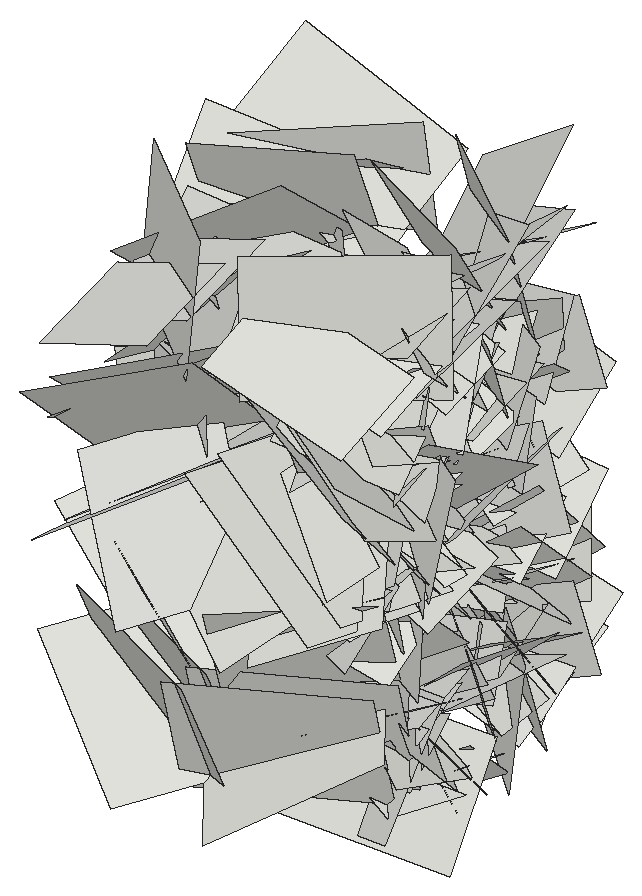
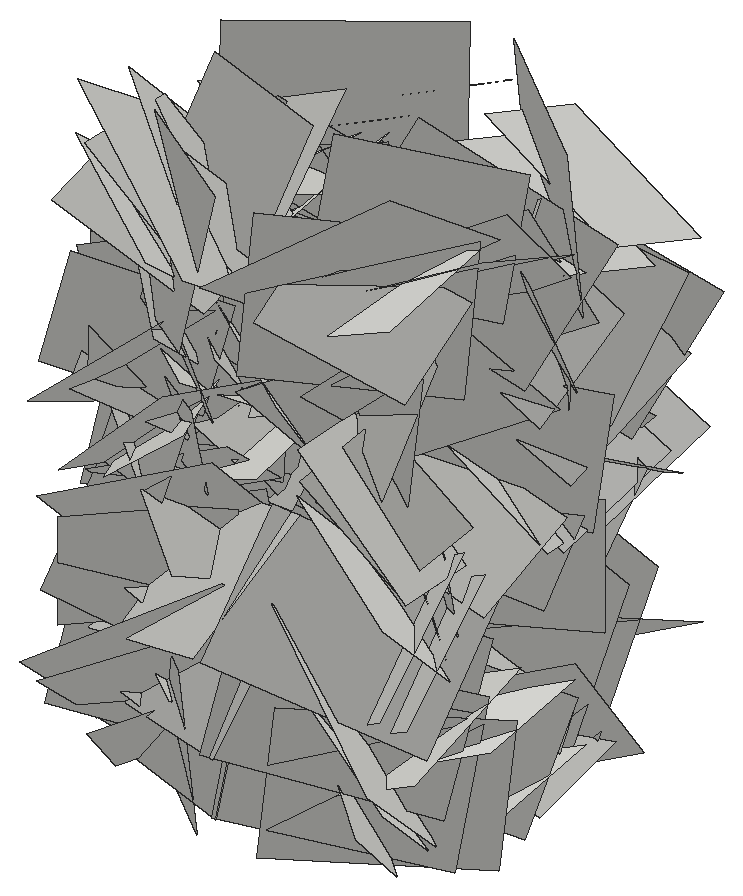
# SketchUp Ruby script. Lengths in inches.
U = 1.inch
M = Sketchup.active_model
def pt(a) = Geom::Point3d.new(a.map { |v| v * U })
def face(e, loops, mat)
  f = e.add_face(loops[0].map { |a| pt(a) })
  loops[1..].each { |l| e.add_face(l.map { |a| pt(a) }).erase! }
  f.material = f.back_material = mat if mat
  f
end
# faces: each face lists its corners as indices into pts; further lists are holes
def faces(e, pts, list, mat = nil) = list.each { |f| face(e, (f[0].is_a?(Array) ? f : [f]).map { |l| l.map { |i| pts[i] } }, mat) }
# xy, xz, yz: faces in a plane at the given z, y or x. An outline is a flat list of corners, or four numbers for a rectangle; further outlines are holes
def ring(l) = l.size == 4 ? [[l[0], l[1]], [l[2], l[1]], [l[2], l[3]], [l[0], l[3]]] : l.each_slice(2).to_a
def flat(e, list, mat, &to3) = list.each { |f| face(e, (f[0].is_a?(Array) ? f : [f]).map { |l| ring(l).map { |u, v| to3.(u, v) } }, mat) }
def xy(e, z, list, mat = nil) = flat(e, list, mat) { |x, y| [x, y, z] }
def xz(e, y, list, mat = nil) = flat(e, list, mat) { |x, z| [x, y, z] }
def yz(e, x, list, mat = nil) = flat(e, list, mat) { |y, z| [x, y, z] }
def lines(e, pts, list) = list.each { |a, b| e.add_line(pt(pts[a]), pt(pts[b])) }
# prism: a flat outline (further loops are holes) pulled along v
def prism(e, loops, v, mat = nil)
  f = face(e, loops, mat); d = Geom::Vector3d.new(v.map { |x| x * U })
  f.pushpull(f.normal.samedirection?(d) ? d.length : -d.length)
end
def box(e, o, s, mat = nil) = prism(e, [[o, [o[0] + s[0], o[1], o[2]], [o[0] + s[0], o[1] + s[1], o[2]], [o[0], o[1] + s[1], o[2]]]], [0, 0, s[2]], mat)
def at(x, y, z, deg = 0) = Geom::Transformation.translation(pt([x, y, z])) * Geom::Transformation.rotation(ORIGIN, Z_AXIS, deg.degrees)
def axes(o, x, y, z) = Geom::Transformation.new([*x, 0, *y, 0, *z, 0, *pt(o).to_a, 1])
def part(name) = M.definitions.add(name)
# library, detail: a bought-in or finely detailed component or shape, given as its bounding box
def library(name, o, s) = part(name).tap { |d| box(d.entities, o, s) }
def detail(e, o, s) = box(e.add_group.entities, o, s)
def put(e, d, t, mat = nil) = e.add_instance(d, t).tap { |i| i.material = mat if mat }
def group(e, t, mat = nil) = e.add_group.tap { |g| g.transformation = t; g.material = mat if mat }.entities
root = M.entities
c1 = part("Component\#6")
p = [[0.01,0,0],[0,3.24,4.54],[4.32,3.24,4.54],[4.33,0,0]]
faces(c1.entities,p,[[0,1,2,3]])
put(root,c1,axes([14.53,133.2,0.29],[-0.16868,0.00753,1.30134],[-0.16064,1.302,-0.02607],[1.37005,0.15359,0.15716]))
put(root,c1,axes([18.5,127.28,0.51],[0.04452,-0.40985,0.5808],[0.07759,0.58122,0.40485],[-0.7495,0.03582,0.07641]))
put(root,c1,axes([14.53,129.68,16.21],[0.16446,-0.17941,-0.82447],[0.07006,-0.83314,0.19373],[0.89165,0.09856,0.13685]))
put(root,c1,axes([18.5,134.26,15.51],[0.13639,0.72841,-0.25059],[0.07067,-0.26364,-0.7321],[-0.81346,0.09922,-0.10562]))
put(root,c1,axes([14.53,128.87,2.92],[0.01411,0.95221,-0.19006],[0.11482,-0.19035,-0.94606],[1.02282,0.00823,0.10882]))
put(root,c1,axes([14.53,138.97,11.375],[-0.02639,-0.72989,-0.72722],[0.07911,-0.7268,0.72691],[1.08928,0.0351,-0.07041]))
put(root,c1,axes([14.53,131.74,20.5625],[-0.11289,-0.41624,-1.03402],[0.06809,-1.03929,0.41174],[1.17957,0.02016,-0.12272]))
put(root,c1,axes([18.5,131.9,7.66],[0.03371,0.19161,0.61883],[0.06203,0.6162,-0.1938],[-0.68388,0.06533,0.01292]))
put(root,c1,axes([14.53,134.95,12.42],[0.03363,0.92541,-1.00089],[-0.39451,-0.95725,-0.89685],[1.39004,-0.29406,-0.23032]))
put(root,c1,axes([18.5,131.8,8.64],[0.08497,0.05507,0.67491],[0.04101,0.67814,-0.05993],[-0.71661,0.04534,0.0766]))
put(root,c1,axes([14.53,137.89,18.97],[0.02244,-0.79516,0.48934],[0.22215,0.48102,0.77258],[0.96443,-0.0923,-0.18934]))
put(root,c1,axes([14.53,137.87,11.82],[0.23548,-0.98581,-0.19043],[-0.17104,-0.22756,0.98976],[1.05044,0.18394,0.20385]))
put(root,c1,axes([14.53,129.625,19.87],[-0.14331,0.9196,0.97349],[-0.15794,0.96203,-0.92947],[1.41069,0.20113,-0.00516]))
put(root,c1,axes([14.53,130.99,8.6],[0.04494,-0.64922,0.68663],[0.20873,0.6783,0.62918],[0.97967,-0.11474,-0.16555]))
put(root,c1,axes([14.53,133.91,11.1875],[-0.02059,0.92356,-0.8814],[-0.20413,-0.87353,-0.91107],[1.33776,-0.11908,-0.15259]))
put(root,c1,axes([14.53,128.56,10.3125],[-0.23413,0.04823,1.24691],[0.1221,1.26168,-0.02839],[1.31707,-0.10839,0.22429]))
put(root,c1,axes([14.53,131.94,16.85],[-0.08825,-0.96476,0.81898],[-0.08011,0.82307,0.9619],[1.33903,-0.01434,0.11152]))
put(root,c1,axes([14.53,131.18,15.16],[0.15294,-1.16278,0.39158],[-0.28955,0.35393,1.15166],[1.26792,0.22109,0.21577]))
put(root,c1,axes([18.5,134.77,2.57],[0.05447,0.40704,0.46107],[0.08155,0.45478,-0.41007],[-0.64681,0.09162,-0.01288]))
put(root,c1,axes([14.53,134.14,22.88],[0.03825,0.99518,-0.25742],[0.13842,-0.25993,-0.98657],[1.08078,-0.00193,0.13547]))
put(root,c1,axes([13.82,124.93,11.12],[0.54058,0.75668,0.32998],[0.30141,0.20311,-0.90522],[0.82148,-0.57246,0.11499]))
put(root,c1,axes([14.53,127.92,6.47],[-0.03611,0.05394,1.13531],[0.09971,1.13206,-0.05096],[1.20066,-0.09239,0.03838]))
put(root,c1,axes([18.5,138.1,17.99],[0.00934,-0.49027,-0.41508],[0.1892,-0.3969,0.47259],[-0.65411,-0.1218,0.13076]))
put(root,c1,axes([14.53,127.69,20.12],[-0.02742,-1.01137,-0.35231],[0.21232,-0.35076,0.99222],[1.1152,0.04191,-0.19757]))
put(root,c1,axes([14.53,130,20.12],[-0.02742,-1.01137,-0.35231],[0.21232,-0.35076,0.99222],[1.1152,0.04191,-0.19757]))
put(root,c1,axes([18.5,129.35,18.22],[0.07955,-0.40219,0.442],[0.06566,0.44831,0.39741],[-0.63004,-0.00406,0.09723]))
put(root,c1,axes([14.53,129.81,24.32],[-0.08615,-0.07511,-1.33483],[-0.12267,-1.33188,0.08199],[1.41184,-0.12031,-0.07433]))
put(root,c1,axes([14.53,131.16,1.32],[0.11103,-1.00768,0.14491],[0.13016,0.15712,1.00381],[1.07125,0.08535,-0.13699]))
put(root,c1,axes([14.53,136.29,19.65],[0.239,0.33681,-1.04778],[-0.13934,-1.05364,-0.36698],[1.15826,-0.19625,0.17205]))
put(root,c1,axes([14.53,129.42,5.47],[-0.26825,1.30607,0.06413],[0.25565,0.11082,-1.30519],[1.36232,0.23638,0.25756]))
put(root,c1,axes([14.53,126.61,12.8],[-0.1414,-0.87971,0.87765],[0.19082,0.8597,0.88908],[1.30331,-0.22132,-0.03495]))
put(root,c1,axes([14.53,133.96,9.66],[0.06967,-1.04066,0.34132],[0.1454,0.34706,1.03175],[1.15177,0.01914,-0.15089]))
put(root,c1,axes([14.53,134.94,17.85],[0.08672,-0.29938,1.1859],[-0.04442,1.18717,0.30259],[1.29573,0.06074,-0.069]))
put(root,c1,axes([14.53,129.48,20.64],[-0.14207,1.22324,0.51937],[0.11373,0.53026,-1.2212],[1.40407,0.08082,0.15147]))
put(root,c1,axes([14.53,129.66,12.47],[-0.1081,-1.2535,0.58167],[-0.00417,0.58351,1.25678],[1.46479,-0.09085,0.0465]))
put(root,c1,axes([14.53,125.82,11.42],[0.20547,0.4933,-0.99975],[0.03886,-1.01702,-0.49472],[1.18108,-0.05236,0.1902]))
put(root,c1,axes([14.53,131.95,0.87],[0.07095,-0.70744,0.83659],[0.30432,0.82019,0.6706],[1.12076,-0.17792,-0.23504]))
put(root,c1,axes([14.53,139.8125,5.82],[0.12038,-0.94885,-0.86303],[-0.08352,-0.86993,0.94607],[1.35702,0.03063,0.13479]))
put(root,c1,axes([14.53,133.04,19.75],[0.14526,-0.49923,0.95494],[0.24012,0.95446,0.46647],[1.11669,-0.1403,-0.22453]))
put(root,c1,axes([14.53,128.24,17.68],[0.22785,0.52614,1.07761],[-0.06777,1.09826,-0.52347],[1.26934,-0.03581,-0.22138]))
put(root,c1,axes([14.53,133.15,22.79],[0.15509,1.06813,0.73269],[-0.10614,0.74447,-1.06531],[1.36888,-0.06329,-0.16562]))
put(root,c1,axes([14.53,132.12,7.08],[-0.00585,1.22451,-0.43101],[0.11167,-0.42917,-1.22063],[1.3715,0.04016,0.09755]))
put(root,c1,axes([14.53,125.99,1.35],[0.00241,0.79041,1.08039],[0.06651,1.07914,-0.78963],[1.41741,-0.05198,0.03522]))
put(root,c1,axes([14.53,127.67,13.74],[0.06329,-0.97705,0.81505],[0.12838,0.8166,0.97005],[1.34259,-0.03203,-0.13118]))
put(root,c1,axes([14.53,137,19.49],[0.23927,-0.1296,-1.18474],[0.04055,-1.20439,0.13904],[1.26266,0.06324,0.22004]))
put(root,c1,axes([14.53,135.39,1.18],[0.01455,-0.40823,1.27358],[0.1801,1.26386,0.40328],[1.40617,-0.15765,-0.06483]))
put(root,c1,axes([14.53,128.0625,10.23],[0.10909,-1.3698,0.20566],[-0.00727,0.20572,1.37363],[1.46824,0.1028,-0.00848]))
put(root,c1,axes([14.53,129.98,10.23],[0.10909,-1.3698,0.20566],[-0.00727,0.20572,1.37363],[1.46824,0.1028,-0.00848]))
put(root,c1,axes([14.53,138.98,4.78],[0.22268,-0.9196,-0.8307],[0.07298,-0.83259,0.9391],[1.31157,0.20246,0.08879]))
put(root,c1,axes([13.36,124.5,5.79],[0.83668,1.07369,0.2523],[0.21003,0.16716,-1.33127],[1.15009,-0.81162,0.05958]))
put(root,c1,axes([14.53,130.78,10.54],[0.24762,-1.26357,-0.1726],[-0.00687,-0.17664,1.28442],[1.3518,0.23056,0.03815]))
put(root,c1,axes([14.53,136.82,5.83],[0.1656,-1.02965,0.80161],[0.14776,0.81588,1.02082],[1.37528,0.03632,-0.2062]))
put(root,c1,axes([14.53,130.15,15.41],[0.24379,0.89731,1.03665],[0.02149,1.04879,-0.91232],[1.45316,-0.16605,-0.16042]))
put(root,c1,axes([14.53,135.96,3.29],[0.1622,-0.76384,1.11136],[0.23079,1.11781,0.7383],[1.4107,-0.09505,-0.24857]))
put(root,c1,axes([14.53,125.3125,7.6875],[0.15543,0.49215,-1.26812],[0.29157,-1.25984,-0.45713],[1.41209,0.20597,0.23397]))
put(root,c1,axes([14.53,126.76,7.6875],[0.15543,0.49215,-1.26812],[0.29157,-1.25984,-0.45713],[1.41209,0.20597,0.23397]))
put(root,c1,axes([14.43,125.5,13.2],[1.07209,0.56535,0.5401],[0.40295,0.41611,-1.14744],[0.72423,-1.06841,-0.1611]))
put(root,c1,axes([28.42,125.5,13.2],[-1.07209,0.56535,0.5401],[-0.40295,0.41611,-1.14744],[-0.72423,-1.06841,-0.1611]))
put(root,c1,axes([28.31,126.76,7.6875],[-0.15543,0.49215,-1.26812],[-0.29157,-1.25984,-0.45713],[-1.41209,0.20597,0.23397]))
put(root,c1,axes([28.31,125.3125,7.6875],[-0.15543,0.49215,-1.26812],[-0.29157,-1.25984,-0.45713],[-1.41209,0.20597,0.23397]))
put(root,c1,axes([28.31,135.96,3.29],[-0.1622,-0.76384,1.11136],[-0.23079,1.11781,0.7383],[-1.4107,-0.09505,-0.24857]))
put(root,c1,axes([28.31,130.15,15.41],[-0.24379,0.89731,1.03665],[-0.02149,1.04879,-0.91232],[-1.45316,-0.16605,-0.16042]))
put(root,c1,axes([28.31,136.82,5.83],[-0.1656,-1.02965,0.80161],[-0.14776,0.81588,1.02082],[-1.37528,0.03632,-0.2062]))
put(root,c1,axes([28.31,130.78,10.54],[-0.24762,-1.26357,-0.1726],[0.00687,-0.17664,1.28442],[-1.3518,0.23056,0.03815]))
put(root,c1,axes([29.48,124.5,5.79],[-0.83668,1.07369,0.2523],[-0.21003,0.16716,-1.33127],[-1.15009,-0.81162,0.05958]))
put(root,c1,axes([28.31,138.98,4.78],[-0.22268,-0.9196,-0.8307],[-0.07298,-0.83259,0.9391],[-1.31157,0.20246,0.08879]))
put(root,c1,axes([28.31,128.0625,10.23],[-0.10909,-1.3698,0.20566],[0.00727,0.20572,1.37363],[-1.46824,0.1028,-0.00848]))
put(root,c1,axes([28.31,129.98,10.23],[-0.10909,-1.3698,0.20566],[0.00727,0.20572,1.37363],[-1.46824,0.1028,-0.00848]))
put(root,c1,axes([28.31,135.39,1.18],[-0.01455,-0.40823,1.27358],[-0.1801,1.26386,0.40328],[-1.40617,-0.15765,-0.06483]))
put(root,c1,axes([28.31,137,19.49],[-0.23927,-0.1296,-1.18474],[-0.04055,-1.20439,0.13904],[-1.26266,0.06324,0.22004]))
put(root,c1,axes([28.31,127.67,13.74],[-0.06329,-0.97705,0.81505],[-0.12838,0.8166,0.97005],[-1.34259,-0.03203,-0.13118]))
put(root,c1,axes([28.31,125.99,1.35],[-0.00241,0.79041,1.08039],[-0.06651,1.07914,-0.78963],[-1.41741,-0.05198,0.03522]))
put(root,c1,axes([28.31,132.12,7.08],[0.00585,1.22451,-0.43101],[-0.11167,-0.42917,-1.22063],[-1.3715,0.04016,0.09755]))
put(root,c1,axes([28.31,133.15,22.79],[-0.15509,1.06813,0.73269],[0.10614,0.74447,-1.06531],[-1.36888,-0.06329,-0.16562]))
put(root,c1,axes([28.31,128.24,17.68],[-0.22785,0.52614,1.07761],[0.06777,1.09826,-0.52347],[-1.26934,-0.03581,-0.22138]))
put(root,c1,axes([28.31,133.04,19.75],[-0.14526,-0.49923,0.95494],[-0.24012,0.95446,0.46647],[-1.11669,-0.1403,-0.22453]))
put(root,c1,axes([28.31,139.8125,5.82],[-0.12038,-0.94885,-0.86303],[0.08352,-0.86993,0.94607],[-1.35702,0.03063,0.13479]))
put(root,c1,axes([28.31,131.95,0.87],[-0.07095,-0.70744,0.83659],[-0.30432,0.82019,0.6706],[-1.12076,-0.17792,-0.23504]))
put(root,c1,axes([28.31,125.82,11.42],[-0.20547,0.4933,-0.99975],[-0.03886,-1.01702,-0.49472],[-1.18108,-0.05236,0.1902]))
put(root,c1,axes([28.31,129.66,12.47],[0.1081,-1.2535,0.58167],[0.00417,0.58351,1.25678],[-1.46479,-0.09085,0.0465]))
put(root,c1,axes([28.31,129.48,20.64],[0.14207,1.22324,0.51937],[-0.11373,0.53026,-1.2212],[-1.40407,0.08082,0.15147]))
put(root,c1,axes([28.31,134.94,17.85],[-0.08672,-0.29938,1.1859],[0.04442,1.18717,0.30259],[-1.29573,0.06074,-0.069]))
put(root,c1,axes([28.31,133.96,9.66],[-0.06967,-1.04066,0.34132],[-0.1454,0.34706,1.03175],[-1.15177,0.01914,-0.15089]))
put(root,c1,axes([28.31,126.61,12.8],[0.1414,-0.87971,0.87765],[-0.19082,0.8597,0.88908],[-1.30331,-0.22132,-0.03495]))
put(root,c1,axes([28.31,129.42,5.47],[0.26825,1.30607,0.06413],[-0.25565,0.11082,-1.30519],[-1.36232,0.23638,0.25756]))
put(root,c1,axes([28.31,136.29,19.65],[-0.239,0.33681,-1.04778],[0.13934,-1.05364,-0.36698],[-1.15826,-0.19625,0.17205]))
put(root,c1,axes([28.31,131.16,1.32],[-0.11103,-1.00768,0.14491],[-0.13016,0.15712,1.00381],[-1.07125,0.08535,-0.13699]))
put(root,c1,axes([28.31,129.81,24.32],[0.08615,-0.07511,-1.33483],[0.12267,-1.33188,0.08199],[-1.41184,-0.12031,-0.07433]))
put(root,c1,axes([24.34,129.35,18.22],[-0.07955,-0.40219,0.442],[-0.06566,0.44831,0.39741],[0.63004,-0.00406,0.09723]))
put(root,c1,axes([28.31,127.69,20.12],[0.02742,-1.01137,-0.35231],[-0.21232,-0.35076,0.99222],[-1.1152,0.04191,-0.19757]))
put(root,c1,axes([28.31,130,20.12],[0.02742,-1.01137,-0.35231],[-0.21232,-0.35076,0.99222],[-1.1152,0.04191,-0.19757]))
put(root,c1,axes([24.34,138.1,17.99],[-0.00934,-0.49027,-0.41508],[-0.1892,-0.3969,0.47259],[0.65411,-0.1218,0.13076]))
put(root,c1,axes([28.31,127.92,6.47],[0.03611,0.05394,1.13531],[-0.09971,1.13206,-0.05096],[-1.20066,-0.09239,0.03838]))
put(root,c1,axes([29.03,124.93,11.12],[-0.54058,0.75668,0.32998],[-0.30141,0.20311,-0.90522],[-0.82148,-0.57246,0.11499]))
put(root,c1,axes([28.31,134.14,22.88],[-0.03825,0.99518,-0.25742],[-0.13842,-0.25993,-0.98657],[-1.08078,-0.00193,0.13547]))
put(root,c1,axes([24.34,134.77,2.57],[-0.05447,0.40704,0.46107],[-0.08155,0.45478,-0.41007],[0.64681,0.09162,-0.01288]))
put(root,c1,axes([28.31,131.18,15.16],[-0.15294,-1.16278,0.39158],[0.28955,0.35393,1.15166],[-1.26792,0.22109,0.21577]))
put(root,c1,axes([28.31,131.94,16.85],[0.08825,-0.96476,0.81898],[0.08011,0.82307,0.9619],[-1.33903,-0.01434,0.11152]))
put(root,c1,axes([28.31,128.56,10.3125],[0.23413,0.04823,1.24691],[-0.1221,1.26168,-0.02839],[-1.31707,-0.10839,0.22429]))
put(root,c1,axes([28.31,133.91,11.1875],[0.02059,0.92356,-0.8814],[0.20413,-0.87353,-0.91107],[-1.33776,-0.11908,-0.15259]))
put(root,c1,axes([28.31,130.99,8.6],[-0.04494,-0.64922,0.68663],[-0.20873,0.6783,0.62918],[-0.97967,-0.11474,-0.16555]))
put(root,c1,axes([28.31,129.625,19.87],[0.14331,0.9196,0.97349],[0.15794,0.96203,-0.92947],[-1.41069,0.20113,-0.00516]))
put(root,c1,axes([28.31,137.87,11.82],[-0.23548,-0.98581,-0.19043],[0.17104,-0.22756,0.98976],[-1.05044,0.18394,0.20385]))
put(root,c1,axes([24.34,131.8,8.64],[-0.08497,0.05507,0.67491],[-0.04101,0.67814,-0.05993],[0.71661,0.04534,0.0766]))
put(root,c1,axes([28.31,134.95,12.42],[-0.03363,0.92541,-1.00089],[0.39451,-0.95725,-0.89685],[-1.39004,-0.29406,-0.23032]))
put(root,c1,axes([24.34,131.9,7.66],[-0.03371,0.19161,0.61883],[-0.06203,0.6162,-0.1938],[0.68388,0.06533,0.01292]))
put(root,c1,axes([28.31,131.74,20.5625],[0.11289,-0.41624,-1.03402],[-0.06809,-1.03929,0.41174],[-1.17957,0.02016,-0.12272]))
put(root,c1,axes([28.31,138.97,11.375],[0.02639,-0.72989,-0.72722],[-0.07911,-0.7268,0.72691],[-1.08928,0.0351,-0.07041]))
put(root,c1,axes([28.31,128.87,2.92],[-0.01411,0.95221,-0.19006],[-0.11482,-0.19035,-0.94606],[-1.02282,0.00823,0.10882]))
put(root,c1,axes([24.34,134.26,15.51],[-0.13639,0.72841,-0.25059],[-0.07067,-0.26364,-0.7321],[0.81346,0.09922,-0.10562]))
put(root,c1,axes([28.31,129.68,16.21],[-0.16446,-0.17941,-0.82447],[-0.07006,-0.83314,0.19373],[-0.89165,0.09856,0.13685]))
put(root,c1,axes([24.34,127.28,0.51],[-0.04452,-0.40985,0.5808],[-0.07759,0.58122,0.40485],[0.7495,0.03582,0.07641]))
put(root,c1,axes([28.31,133.2,0.29],[0.16868,0.00753,1.30134],[0.16064,1.302,-0.02607],[-1.37005,0.15359,0.15716]))
put(root,c1,axes([24.34,134.57,7.51],[-0.06425,-0.0713,-0.65597],[0.02618,-0.65852,0.06929],[0.69893,0.01811,-0.0629]))
put(root,c1,axes([28.31,128.52,17.74],[-0.08604,0.43028,-0.81229],[-0.04293,-0.81633,-0.42838],[-0.97342,-0.00203,0.0907]))
put(root,c1,axes([24.34,132.11,13.83],[-0.12823,-0.67114,-0.46171],[-0.10246,-0.45164,0.68184],[0.85739,-0.15435,0.01243]))
put(root,c1,axes([28.31,133.79,15.82],[-0.11741,-0.82822,-0.37202],[-0.00882,-0.37384,0.83474],[-0.96237,0.10447,0.03774]))
put(root,c1,axes([24.34,131.53,3.64],[-0.03356,0.34972,-0.55611],[0.01458,-0.55628,-0.35061],[0.69619,0.02851,-0.01946]))
put(root,c1,axes([24.34,130.57,14.69],[-0.08088,0.56373,-0.36339],[0.06437,-0.35843,-0.56878],[0.70803,0.09698,0.0102]))
put(root,c1,axes([28.31,130.125,12.36],[0.14413,1.23778,0.56401],[0.30073,0.52855,-1.22835],[-1.41013,0.23923,-0.20431]))
put(root,c1,axes([28.31,129.28,18.375],[-0.15104,-0.37703,-0.77667],[0.00911,-0.78776,0.38083],[-0.9151,0.05438,0.13199]))
put(root,c1,axes([28.31,132.6,22.9],[-0.05818,0.99288,0.05669],[0.07779,0.06066,-0.99145],[-1.05129,-0.05046,-0.07649]))
put(root,c1,axes([24.34,133.3125,17.59],[0.01529,0.27468,0.5349],[0.08187,0.52978,-0.27413],[0.6321,-0.07526,0.02257]))
put(root,c1,axes([24.34,129.84,16.13],[0.05288,0.68465,0.04631],[-0.09068,0.05228,-0.68068],[0.72171,-0.04359,-0.08892]))
put(root,c1,axes([28.31,129.45,15.69],[0.00555,0.72683,0.86308],[0.19522,0.85097,-0.71774],[-1.18002,0.1442,-0.11468]))
put(root,c1,axes([24.34,129.41,10.95],[-0.18775,-0.48629,-0.69123],[0.00245,-0.70652,0.49646],[0.89586,-0.09998,-0.14623]))
put(root,c1,axes([24.34,132.63,6.14],[-0.10731,0.87556,-0.00554],[-0.12201,-0.01884,-0.87366],[0.92006,0.09962,-0.1165]))
put(root,c1,axes([28.31,133.96,12.5],[-0.03937,0.24323,0.81298],[-0.12274,0.80469,-0.24604],[-0.89109,-0.12158,-0.00203]))
put(root,c1,axes([28.31,127.6,6.32],[-0.09105,0.77875,-0.27248],[-0.08108,-0.28029,-0.77696],[-0.87078,-0.05533,0.10084]))
put(root,c1,axes([28.31,133.1,9.3125],[0.02086,0.87239,-0.16813],[-0.14049,-0.16341,-0.8634],[-0.93122,0.04419,0.12649]))
put(root,c1,axes([28.31,131.05,1.96],[0.03915,-1.05631,0.36623],[0.17317,0.36759,1.04378],[-1.17236,0.01903,0.16641]))
put(root,c1,axes([24.34,133.88,6.93],[-0.12434,-0.60409,0.41763],[0.12699,0.40152,0.61444],[0.76804,-0.16419,-0.03398]))
put(root,c1,axes([28.31,136.93,7.59],[0.11136,0.24127,-0.97313],[-0.07388,-0.97433,-0.24909],[-1.06018,0.09324,-0.08486]))
put(root,c1,axes([24.34,130.03,2.94],[-0.11679,-0.3481,0.76621],[-0.04914,0.77408,0.34502],[0.89071,-0.00294,0.1195]))
put(root,c1,axes([24.34,129.23,5.41],[-0.17398,-0.60139,0.60701],[0.02487,0.6147,0.61536],[0.9054,-0.13245,0.09973]))
put(root,c1,axes([28.31,132.5,3.06],[0.12033,-0.77552,-0.96336],[0.26418,-0.93322,0.78062],[-1.28404,-0.26468,0.07033]))
put(root,c1,axes([24.34,129.18,10.77],[0.08644,0.04023,-0.60323],[0.06997,-0.60565,-0.03147],[0.63702,0.06107,0.08531]))
put(root,c1,axes([28.31,132.55,10.48],[0.11298,-1.07137,-0.22101],[0.09706,-0.21254,1.07447],[-1.1555,-0.12261,0.06864]))
put(root,c1,axes([24.34,128.34,18.92],[0.04874,0.38349,0.62334],[-0.06251,0.62448,-0.37984],[0.77325,0.02631,-0.07]))
put(root,c1,axes([24.34,129.8,15.91],[0.05085,-0.71724,0.33006],[-0.13843,0.31891,0.71198],[0.82538,0.09767,0.09907]))
put(root,c1,axes([28.31,127.86,19.19],[0.25173,1.01088,0.57921],[0.04385,0.58343,-1.03521],[-1.23418,0.22691,0.08136]))
put(root,c1,axes([28.31,127.34,21.1],[0.03089,0.79811,0.32897],[-0.11706,0.3299,-0.79059],[-0.90753,-0.01539,0.11317]))
put(root,c1,axes([24.34,133.42,16.97],[-0.14677,0.94615,0.46149],[-0.22557,0.4307,-0.94687],[1.09283,0.21597,-0.13346]))
put(root,c1,axes([24.34,133.96,6.46],[-0.0893,0.11056,0.97068],[-0.19494,0.95507,-0.12474],[1.01706,0.19277,0.06132]))
put(root,c1,axes([28.31,136.53,11.26],[0.01536,-0.64622,-0.54667],[-0.11065,-0.54394,0.64022],[-0.89037,0.05645,-0.089]))
put(root,c1,axes([24.34,131.99,-0.9375],[0.0225,-0.54484,0.50649],[-0.02225,0.50605,0.54525],[0.78821,0.02984,0.00093]))
put(root,c1,axes([28.31,127.95,5.4],[-0.05879,0.74539,0.22064],[-0.10629,0.21249,-0.74307],[-0.81711,-0.08127,0.08079]))
put(root,c1,axes([24.34,125.86,8.82],[0.02658,0.53015,0.39509],[0.11889,0.38623,-0.52538],[0.69069,-0.08688,0.07523]))
put(root,c1,axes([24.34,131.86,3.01],[0.01467,-0.55248,-0.51034],[-0.00827,-0.51051,0.55244],[0.7972,0.00487,0.01512]))
put(root,c1,axes([24.34,136.82,15.87],[-0.16772,-0.74319,-0.48228],[0.03783,-0.49486,0.75087],[0.93836,-0.11289,-0.11647]))
put(root,c1,axes([28.31,125.93,11.7],[-0.16945,0.67455,-0.05214],[-0.09647,-0.07453,-0.68517],[-0.71064,-0.15073,0.10544]))
put(root,c1,axes([28.31,127.92,4.7],[-0.092,0.70183,0.2556],[-0.07294,0.24871,-0.70628],[-0.78837,-0.10491,0.03552]))
put(root,c1,axes([28.31,128.53,16.93],[0.30517,1.08519,-0.55956],[0.1011,-0.59314,-1.10124],[-1.29027,0.21019,-0.21864]))
put(root,c1,axes([24.34,137.37,4.77],[-0.01509,-0.67708,-0.46908],[-0.05072,-0.46768,0.67651],[0.87164,-0.03894,0.03124]))
put(root,c1,axes([28.31,133.14,16.06],[0.03738,-0.31853,0.81486],[-0.04959,0.81367,0.32009],[-0.92608,-0.05642,0.01575]))
put(root,c1,axes([28.31,133.58,20.74],[0.06025,0.71815,0.57437],[0.00066,0.57544,-0.71955],[-0.97476,0.04478,0.03501]))
put(root,c1,axes([28.31,131.35,15.19],[-0.02447,0.82058,-0.14823],[-0.01236,-0.14859,-0.82075],[-0.8838,-0.02064,0.01558]))
put(root,c1,axes([24.34,130.01,4.69],[0.05447,0.12092,0.77662],[-0.06993,0.77619,-0.11649],[0.83019,0.05744,-0.06077]))
put(root,c1,axes([28.31,135.14,15.06],[0.15738,0.18416,-1.10832],[0.16264,-1.1108,-0.16402],[-1.17977,-0.12857,-0.17046]))
put(root,c1,axes([28.31,133.07,14.74],[0.12706,0.28525,0.91315],[-0.02767,0.92092,-0.28425],[-1.01369,0.01061,0.12222]))
put(root,c1,axes([28.31,132.96,18.89],[0.10145,-0.91774,-0.17179],[-0.02227,-0.17476,0.92192],[-0.98945,-0.09016,-0.03837]))
put(root,c1,axes([24.34,135.65,2.32],[-0.1935,-1.06071,0.09437],[-0.13048,0.11613,1.0671],[1.12123,-0.16954,0.14047]))
put(root,c1,axes([24.34,136.42,13.64],[0.14309,-0.55174,0.41683],[-0.03038,0.41987,0.56505],[0.73236,0.12522,-0.058]))
put(root,c1,axes([28.31,137.27,19.36],[0.1763,0.15017,-0.9005],[-0.15684,-0.89878,-0.17721],[-0.95491,0.17535,-0.13715]))
put(root,c1,axes([28.31,130.2,1.79],[0.1042,-0.77086,0.73803],[0.17604,0.74317,0.75412],[-1.11745,0.04519,0.18762]))
put(root,c1,axes([28.31,136.01,11.51],[-0.06598,-0.27091,0.62957],[-0.16839,0.62065,0.25136],[-0.70672,-0.12259,-0.11867]))
put(root,c1,axes([24.34,133.51,8.98],[-0.15319,0.47062,-0.90401],[-0.09722,-0.91536,-0.46187],[1.07594,-0.0157,-0.17044]))
put(root,c1,axes([28.31,126.24,11.02],[-0.17433,0.41563,0.4957],[-0.04437,0.50356,-0.43611],[-0.68427,-0.13854,-0.09801]))
